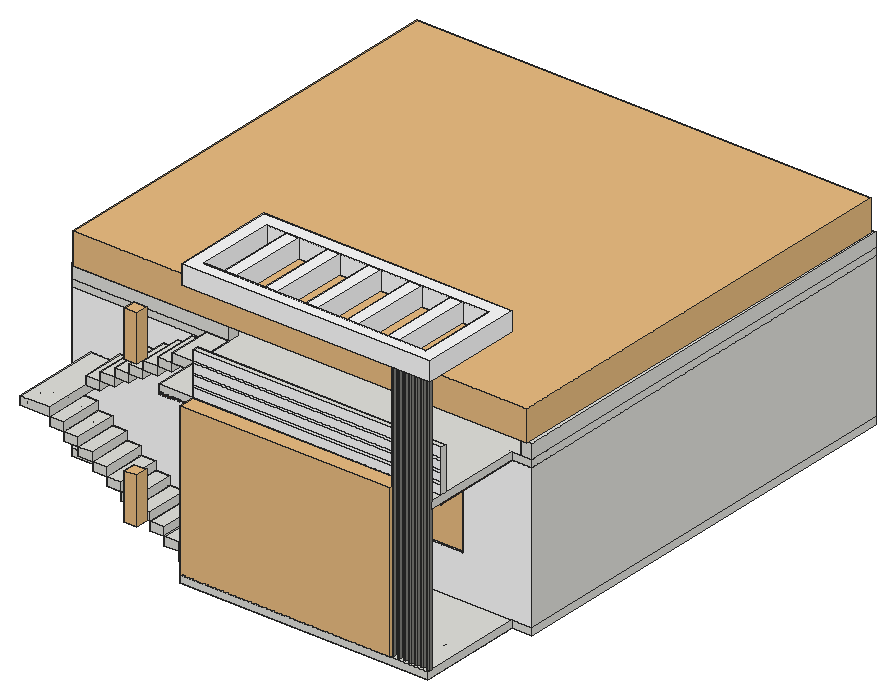
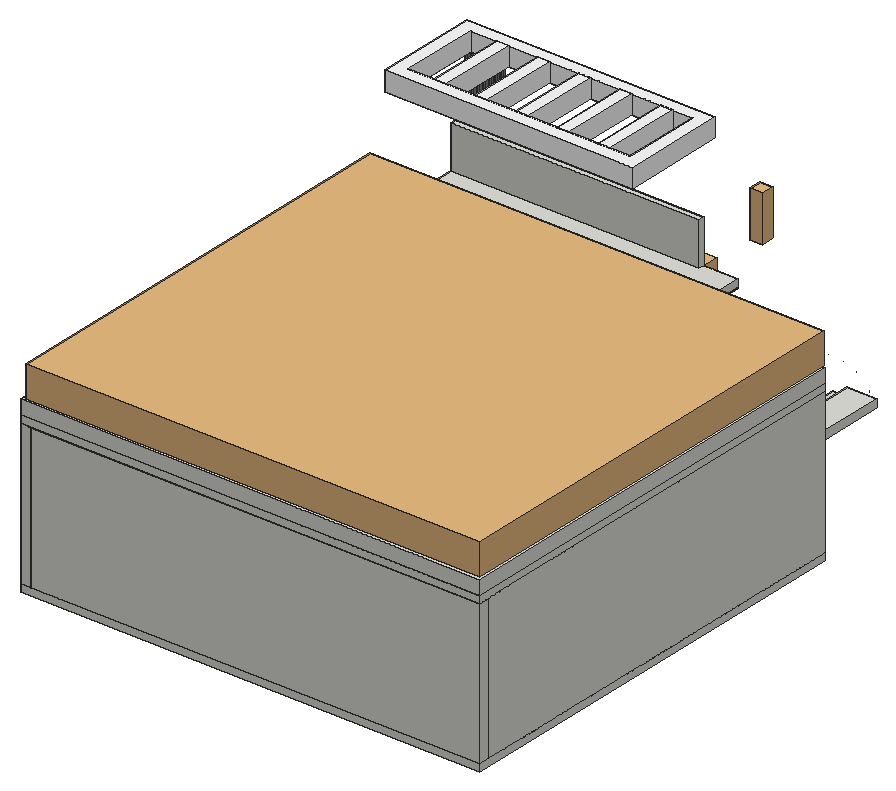
# SketchUp Ruby script. Lengths in inches.
U = 1.inch
M = Sketchup.active_model
def pt(a) = Geom::Point3d.new(a.map { |v| v * U })
def face(e, loops, mat)
  f = e.add_face(loops[0].map { |a| pt(a) })
  loops[1..].each { |l| e.add_face(l.map { |a| pt(a) }).erase! }
  f.material = f.back_material = mat if mat
  f
end
# faces: each face lists its corners as indices into pts; further lists are holes
def faces(e, pts, list, mat = nil) = list.each { |f| face(e, (f[0].is_a?(Array) ? f : [f]).map { |l| l.map { |i| pts[i] } }, mat) }
# xy, xz, yz: faces in a plane at the given z, y or x. An outline is a flat list of corners, or four numbers for a rectangle; further outlines are holes
def ring(l) = l.size == 4 ? [[l[0], l[1]], [l[2], l[1]], [l[2], l[3]], [l[0], l[3]]] : l.each_slice(2).to_a
def flat(e, list, mat, &to3) = list.each { |f| face(e, (f[0].is_a?(Array) ? f : [f]).map { |l| ring(l).map { |u, v| to3.(u, v) } }, mat) }
def xy(e, z, list, mat = nil) = flat(e, list, mat) { |x, y| [x, y, z] }
def xz(e, y, list, mat = nil) = flat(e, list, mat) { |x, z| [x, y, z] }
def yz(e, x, list, mat = nil) = flat(e, list, mat) { |y, z| [x, y, z] }
def lines(e, pts, list) = list.each { |a, b| e.add_line(pt(pts[a]), pt(pts[b])) }
# prism: a flat outline (further loops are holes) pulled along v
def prism(e, loops, v, mat = nil)
  f = face(e, loops, mat); d = Geom::Vector3d.new(v.map { |x| x * U })
  f.pushpull(f.normal.samedirection?(d) ? d.length : -d.length)
end
def box(e, o, s, mat = nil) = prism(e, [[o, [o[0] + s[0], o[1], o[2]], [o[0] + s[0], o[1] + s[1], o[2]], [o[0], o[1] + s[1], o[2]]]], [0, 0, s[2]], mat)
def at(x, y, z, deg = 0) = Geom::Transformation.translation(pt([x, y, z])) * Geom::Transformation.rotation(ORIGIN, Z_AXIS, deg.degrees)
def axes(o, x, y, z) = Geom::Transformation.new([*x, 0, *y, 0, *z, 0, *pt(o).to_a, 1])
def part(name) = M.definitions.add(name)
# library, detail: a bought-in or finely detailed component or shape, given as its bounding box
def library(name, o, s) = part(name).tap { |d| box(d.entities, o, s) }
def detail(e, o, s) = box(e.add_group.entities, o, s)
def put(e, d, t, mat = nil) = e.add_instance(d, t).tap { |i| i.material = mat if mat }
def group(e, t, mat = nil) = e.add_group.tap { |g| g.transformation = t; g.material = mat if mat }.entities
root = M.entities
M.materials.add("Carpaint Black Matte 1.5cm").color = [255, 255, 255]
M.materials.add("Ecorel - epc61025 33.57cm").color = [255, 255, 255]
M.materials.add("Iron Rough 15cm").color = [129, 129, 125]
M.materials.add("Leather Brown Alcantara 004 9.18cm").color = [255, 255, 255]
M.materials.add("Pp-1846-msg 17.72cm").color = [255, 255, 255]
M.materials.add("Wood Mahogany 33-46 100cm").color = [84, 42, 21]
M.materials.add("XPS Yellow SSS 1.51cm\#2").color = [255, 255, 255]
c1 = part("Group231\#1")
box(c1.entities,[-103.625,-42.25,0],[2,84.5,2])
c2 = part("Group232\#1")
box(c2.entities,[-99.625,-42.25,0],[2,84.5,2])
c3 = part("Group233\#1")
box(c3.entities,[-95.625,-42.25,0],[2,84.5,2])
c4 = part("Group234\#1")
box(c4.entities,[-91.625,-42.25,0],[2,84.5,2])
c5 = part("Group235\#1")
box(c5.entities,[-87.625,-42.25,0],[2,84.5,2])
c6 = part("Group236\#1")
box(c6.entities,[-83.625,-42.25,0],[2,84.5,2])
c7 = part("Group237\#1")
box(c7.entities,[-79.625,-42.25,0],[2,84.5,2])
c8 = part("Group238\#1")
box(c8.entities,[-75.625,-42.25,0],[2,84.5,2])
c9 = part("Group239\#1")
box(c9.entities,[-71.625,-42.25,0],[2,84.5,2])
c10 = part("Group240\#1")
box(c10.entities,[-67.625,-42.25,0],[2,84.5,2])
c11 = part("Group241\#1")
box(c11.entities,[-63.625,-42.25,0],[2,84.5,2])
c12 = part("Group242\#1")
box(c12.entities,[-59.625,-42.25,0],[2,84.5,2])
c13 = part("Group243\#1")
box(c13.entities,[-55.625,-42.25,0],[2,84.5,2])
c14 = part("Group244\#1")
box(c14.entities,[-51.625,-42.25,0],[2,84.5,2])
c15 = part("Group245\#1")
box(c15.entities,[-47.625,-42.25,0],[2,84.5,2])
c16 = part("Group246\#1")
box(c16.entities,[-43.625,-42.25,0],[2,84.5,2])
c17 = part("Group247\#1")
box(c17.entities,[-39.625,-42.25,0],[2,84.5,2])
c18 = part("Group248\#1")
box(c18.entities,[-35.625,-42.25,0],[2,84.5,2])
c19 = part("Group249\#1")
box(c19.entities,[-31.625,-42.25,0],[2,84.5,2])
c20 = part("Group250\#1")
box(c20.entities,[-27.625,-42.25,0],[2,84.5,2])
c21 = part("Group251\#1")
box(c21.entities,[-23.625,-42.25,0],[2,84.5,2])
c22 = part("Group252\#1")
box(c22.entities,[-19.625,-42.25,0],[2,84.5,2])
c23 = part("Group253\#1")
box(c23.entities,[-15.625,-42.25,0],[2,84.5,2])
c24 = part("Group254\#1")
box(c24.entities,[-11.625,-42.25,0],[2,84.5,2])
c25 = part("Group255\#1")
box(c25.entities,[-7.625,-42.25,0],[2,84.5,2])
c26 = part("Group256\#1")
box(c26.entities,[-3.625,-42.25,0],[2,84.5,2])
c27 = part("Group257\#1")
xy(c27.entities,0,[[0.375,-42.25,0.375,-42.1,2.375,-41.28,2.375,-42.25],[0.375,-42.1,0.375,42.25,2.375,42.25,2.375,-41.28]])
xy(c27.entities,2,[[0.375,-42.25,2.375,42.25]])
xz(c27.entities,-42.25,[[0.375,0,2.375,2]])
xz(c27.entities,42.25,[[0.375,0,2.375,2]])
yz(c27.entities,0.375,[[-42.25,0,42.25,2]])
yz(c27.entities,2.375,[[-42.25,0,42.25,2]])
c28 = part("Group258\#1")
xy(c28.entities,0,[[4.375,-42.25,4.375,-40.47,6.375,-39.65,6.375,-42.25],[4.375,-40.47,4.375,42.25,6.375,42.25,6.375,-39.65]])
xy(c28.entities,2,[[4.375,-42.25,6.375,42.25]])
xz(c28.entities,-42.25,[[4.375,0,6.375,2]])
xz(c28.entities,42.25,[[4.375,0,6.375,2]])
yz(c28.entities,4.375,[[-42.25,0,42.25,2]])
yz(c28.entities,6.375,[[-42.25,0,42.25,2]])
c29 = part("Group259\#1")
xy(c29.entities,0,[[8.375,-42.25,8.375,-38.84,10.375,-38.02,10.375,-42.25],[8.375,-38.84,8.375,42.25,10.375,42.25,10.375,-38.02]])
xy(c29.entities,2,[[8.375,-42.25,10.375,42.25]])
xz(c29.entities,-42.25,[[8.375,0,10.375,2]])
xz(c29.entities,42.25,[[8.375,0,10.375,2]])
yz(c29.entities,8.375,[[-42.25,0,42.25,2]])
yz(c29.entities,10.375,[[-42.25,0,42.25,2]])
c30 = part("Group260\#1")
xy(c30.entities,0,[[12.375,-42.25,12.375,-37.2,14.375,-36.39,14.375,-42.25],[12.375,-37.2,12.375,42.25,14.375,42.25,14.375,-36.39]])
xy(c30.entities,2,[[12.375,-42.25,14.375,42.25]])
xz(c30.entities,-42.25,[[12.375,0,14.375,2]])
xz(c30.entities,42.25,[[12.375,0,14.375,2]])
yz(c30.entities,12.375,[[-42.25,0,42.25,2]])
yz(c30.entities,14.375,[[-42.25,0,42.25,2]])
c31 = part("Group261\#1")
xy(c31.entities,0,[[16.375,-42.25,16.375,-35.57,18.375,-34.76,18.375,-42.25],[16.375,-35.57,16.375,42.25,18.375,42.25,18.375,-34.76]])
xy(c31.entities,2,[[16.375,-42.25,18.375,42.25]])
xz(c31.entities,-42.25,[[16.375,0,18.375,2]])
xz(c31.entities,42.25,[[16.375,0,18.375,2]])
yz(c31.entities,16.375,[[-42.25,0,42.25,2]])
yz(c31.entities,18.375,[[-42.25,0,42.25,2]])
c32 = part("Group262\#1")
xy(c32.entities,0,[[20.375,-42.25,20.375,-33.94,22.375,-33.13,22.375,-42.25],[20.375,-33.94,20.375,42.25,22.375,42.25,22.375,-33.13]])
xy(c32.entities,2,[[20.375,-42.25,22.375,42.25]])
xz(c32.entities,-42.25,[[20.375,0,22.375,2]])
xz(c32.entities,42.25,[[20.375,0,22.375,2]])
yz(c32.entities,20.375,[[-42.25,0,42.25,2]])
yz(c32.entities,22.375,[[-42.25,0,42.25,2]])
c33 = part("Group263\#1")
xy(c33.entities,0,[[24.375,-42.25,24.375,-32.3125,26.375,-31.5,26.375,-42.25],[24.375,-32.3125,24.375,42.25,26.375,42.25,26.375,-31.5]])
xy(c33.entities,2,[[24.375,-42.25,26.375,42.25]])
xz(c33.entities,-42.25,[[24.375,0,26.375,2]])
xz(c33.entities,42.25,[[24.375,0,26.375,2]])
yz(c33.entities,24.375,[[-42.25,0,42.25,2]])
yz(c33.entities,26.375,[[-42.25,0,42.25,2]])
c34 = part("Group264\#1")
xy(c34.entities,0,[[28.375,-42.25,28.375,-30.68,30.375,-29.87,30.375,-42.25],[28.375,-30.68,28.375,42.25,30.375,42.25,30.375,-29.87]])
xy(c34.entities,2,[[28.375,-42.25,30.375,42.25]])
xz(c34.entities,-42.25,[[28.375,0,30.375,2]])
xz(c34.entities,42.25,[[28.375,0,30.375,2]])
yz(c34.entities,28.375,[[-42.25,0,42.25,2]])
yz(c34.entities,30.375,[[-42.25,0,42.25,2]])
c35 = part("Group265\#1")
xy(c35.entities,0,[[32.375,-42.25,32.375,-29.05,34.375,-28.24,34.375,-42.25],[32.375,-29.05,32.375,42.25,34.375,42.25,34.375,-28.24]])
xy(c35.entities,2,[[32.375,-42.25,34.375,42.25]])
xz(c35.entities,-42.25,[[32.375,0,34.375,2]])
xz(c35.entities,42.25,[[32.375,0,34.375,2]])
yz(c35.entities,32.375,[[-42.25,0,42.25,2]])
yz(c35.entities,34.375,[[-42.25,0,42.25,2]])
c36 = part("Group266\#1")
xy(c36.entities,0,[[36.375,-42.25,36.375,-27.42,38.375,-26.6,38.375,-42.25],[36.375,-27.42,36.375,42.25,38.375,42.25,38.375,-26.6]])
xy(c36.entities,2,[[36.375,-42.25,38.375,42.25]])
xz(c36.entities,-42.25,[[36.375,0,38.375,2]])
xz(c36.entities,42.25,[[36.375,0,38.375,2]])
yz(c36.entities,36.375,[[-42.25,0,42.25,2]])
yz(c36.entities,38.375,[[-42.25,0,42.25,2]])
c37 = part("Group267\#1")
xy(c37.entities,0,[[40.375,-42.25,40.375,-25.79,42.375,-24.97,42.375,-42.25],[40.375,-25.79,40.375,42.25,42.375,42.25,42.375,-24.97]])
xy(c37.entities,2,[[40.375,-42.25,42.375,42.25]])
xz(c37.entities,-42.25,[[40.375,0,42.375,2]])
xz(c37.entities,42.25,[[40.375,0,42.375,2]])
yz(c37.entities,40.375,[[-42.25,0,42.25,2]])
yz(c37.entities,42.375,[[-42.25,0,42.25,2]])
c38 = part("Group268\#1")
xy(c38.entities,0,[[44.375,-42.25,44.375,-24.16,46.375,-23.34,46.375,-42.25],[44.375,-24.16,44.375,42.25,46.375,42.25,46.375,-23.34]])
xy(c38.entities,2,[[44.375,-42.25,46.375,42.25]])
xz(c38.entities,-42.25,[[44.375,0,46.375,2]])
xz(c38.entities,42.25,[[44.375,0,46.375,2]])
yz(c38.entities,44.375,[[-42.25,0,42.25,2]])
yz(c38.entities,46.375,[[-42.25,0,42.25,2]])
c39 = part("Group269\#1")
xy(c39.entities,0,[[48.375,-42.25,48.375,-22.53,50.375,-21.71,50.375,-42.25],[48.375,-22.53,48.375,42.25,50.375,42.25,50.375,-21.71]])
xy(c39.entities,2,[[48.375,-42.25,50.375,42.25]])
xz(c39.entities,-42.25,[[48.375,0,50.375,2]])
xz(c39.entities,42.25,[[48.375,0,50.375,2]])
yz(c39.entities,48.375,[[-42.25,0,42.25,2]])
yz(c39.entities,50.375,[[-42.25,0,42.25,2]])
c40 = part("Group270\#1")
xy(c40.entities,0,[[52.375,-42.25,52.375,-20.9,54.375,-20.08,54.375,-42.25],[52.375,-20.9,52.375,42.25,54.375,42.25,54.375,-20.08]])
xy(c40.entities,2,[[52.375,-42.25,54.375,42.25]])
xz(c40.entities,-42.25,[[52.375,0,54.375,2]])
xz(c40.entities,42.25,[[52.375,0,54.375,2]])
yz(c40.entities,52.375,[[-42.25,0,42.25,2]])
yz(c40.entities,54.375,[[-42.25,0,42.25,2]])
c41 = part("Group271\#1")
xy(c41.entities,0,[[56.375,-42.25,56.375,-19.27,58.375,-18.45,58.375,-42.25],[56.375,-19.27,56.375,42.25,58.375,42.25,58.375,-18.45]])
xy(c41.entities,2,[[56.375,-42.25,58.375,42.25]])
xz(c41.entities,-42.25,[[56.375,0,58.375,2]])
xz(c41.entities,42.25,[[56.375,0,58.375,2]])
yz(c41.entities,56.375,[[-42.25,0,42.25,2]])
yz(c41.entities,58.375,[[-42.25,0,42.25,2]])
c42 = part("Group272\#1")
xy(c42.entities,0,[[60.375,-42.25,60.375,-17.63,62.375,-16.82,62.375,-42.25],[60.375,-17.63,60.375,42.25,62.375,42.25,62.375,-16.82]])
xy(c42.entities,2,[[60.375,-42.25,62.375,42.25]])
xz(c42.entities,-42.25,[[60.375,0,62.375,2]])
xz(c42.entities,42.25,[[60.375,0,62.375,2]])
yz(c42.entities,60.375,[[-42.25,0,42.25,2]])
yz(c42.entities,62.375,[[-42.25,0,42.25,2]])
c43 = part("Group273\#1")
xy(c43.entities,0,[[64.375,-42.25,64.375,-16,66.375,-15.1875,66.375,-42.25],[64.375,-16,64.375,42.25,66.375,42.25,66.375,-15.1875]])
xy(c43.entities,2,[[64.375,-42.25,66.375,42.25]])
xz(c43.entities,-42.25,[[64.375,0,66.375,2]])
xz(c43.entities,42.25,[[64.375,0,66.375,2]])
yz(c43.entities,64.375,[[-42.25,0,42.25,2]])
yz(c43.entities,66.375,[[-42.25,0,42.25,2]])
c44 = part("Group274\#1")
xy(c44.entities,0,[[68.375,-42.25,68.375,-14.37,70.375,-13.56,70.375,-42.25],[68.375,-14.37,68.375,42.25,70.375,42.25,70.375,-13.56]])
xy(c44.entities,2,[[68.375,-42.25,70.375,42.25]])
xz(c44.entities,-42.25,[[68.375,0,70.375,2]])
xz(c44.entities,42.25,[[68.375,0,70.375,2]])
yz(c44.entities,68.375,[[-42.25,0,42.25,2]])
yz(c44.entities,70.375,[[-42.25,0,42.25,2]])
c45 = part("Group275\#1")
xy(c45.entities,0,[[72.375,-42.25,72.375,-12.74,74.375,-11.93,74.375,-42.25],[72.375,-12.74,72.375,42.25,74.375,42.25,74.375,-11.93]])
xy(c45.entities,2,[[72.375,-42.25,74.375,42.25]])
xz(c45.entities,-42.25,[[72.375,0,74.375,2]])
xz(c45.entities,42.25,[[72.375,0,74.375,2]])
yz(c45.entities,72.375,[[-42.25,0,42.25,2]])
yz(c45.entities,74.375,[[-42.25,0,42.25,2]])
c46 = part("Group276\#1")
xy(c46.entities,0,[[76.375,-42.25,76.375,-11.11,78.375,-10.3,78.375,-42.25],[76.375,-11.11,76.375,42.25,78.375,42.25,78.375,-10.3]])
xy(c46.entities,2,[[76.375,-42.25,78.375,42.25]])
xz(c46.entities,-42.25,[[76.375,0,78.375,2]])
xz(c46.entities,42.25,[[76.375,0,78.375,2]])
yz(c46.entities,76.375,[[-42.25,0,42.25,2]])
yz(c46.entities,78.375,[[-42.25,0,42.25,2]])
c47 = part("Group277\#1")
xy(c47.entities,0,[[80.375,-42.25,80.375,-9.48,82.375,-8.66,82.375,-42.25],[80.375,-9.48,80.375,42.25,82.375,42.25,82.375,-8.66]])
xy(c47.entities,2,[[80.375,-42.25,82.375,42.25]])
xz(c47.entities,-42.25,[[80.375,0,82.375,2]])
xz(c47.entities,42.25,[[80.375,0,82.375,2]])
yz(c47.entities,80.375,[[-42.25,0,42.25,2]])
yz(c47.entities,82.375,[[-42.25,0,42.25,2]])
c48 = part("Group278\#1")
xy(c48.entities,0,[[84.375,-42.25,84.375,-7.85,86.375,-7.03,86.375,-42.25],[84.375,-7.85,84.375,42.25,86.375,42.25,86.375,-7.03]])
xy(c48.entities,2,[[84.375,-42.25,86.375,42.25]])
xz(c48.entities,-42.25,[[84.375,0,86.375,2]])
xz(c48.entities,42.25,[[84.375,0,86.375,2]])
yz(c48.entities,84.375,[[-42.25,0,42.25,2]])
yz(c48.entities,86.375,[[-42.25,0,42.25,2]])
c49 = part("Group279\#1")
xy(c49.entities,0,[[88.375,-42.25,88.375,-6.22,90.375,-5.4,90.375,-42.25],[88.375,-6.22,88.375,42.25,90.375,42.25,90.375,-5.4]])
xy(c49.entities,2,[[88.375,-42.25,90.375,42.25]])
xz(c49.entities,-42.25,[[88.375,0,90.375,2]])
xz(c49.entities,42.25,[[88.375,0,90.375,2]])
yz(c49.entities,88.375,[[-42.25,0,42.25,2]])
yz(c49.entities,90.375,[[-42.25,0,42.25,2]])
c50 = part("Group280\#1")
xy(c50.entities,0,[[92.375,-42.25,92.375,-4.59,94.375,-3.77,94.375,-42.25],[92.375,-4.59,92.375,42.25,94.375,42.25,94.375,-3.77]])
xy(c50.entities,2,[[92.375,-42.25,94.375,42.25]])
xz(c50.entities,-42.25,[[92.375,0,94.375,2]])
xz(c50.entities,42.25,[[92.375,0,94.375,2]])
yz(c50.entities,92.375,[[-42.25,0,42.25,2]])
yz(c50.entities,94.375,[[-42.25,0,42.25,2]])
c51 = part("Group281\#1")
xy(c51.entities,0,[[96.375,-42.25,96.375,-2.96,98.375,-2.14,98.375,-42.25],[96.375,-2.96,96.375,42.25,98.375,42.25,98.375,-2.14]])
xy(c51.entities,2,[[96.375,-42.25,98.375,42.25]])
xz(c51.entities,-42.25,[[96.375,0,98.375,2]])
xz(c51.entities,42.25,[[96.375,0,98.375,2]])
yz(c51.entities,96.375,[[-42.25,0,42.25,2]])
yz(c51.entities,98.375,[[-42.25,0,42.25,2]])
c52 = part("Group282\#1")
xy(c52.entities,0,[[100.375,-42.25,100.375,-1.33,102.375,-0.51,102.375,-42.25],[100.375,-1.33,100.375,42.25,102.375,42.25,102.375,-0.51]])
xy(c52.entities,2,[[100.375,-42.25,102.375,42.25]])
xz(c52.entities,-42.25,[[100.375,0,102.375,2]])
xz(c52.entities,42.25,[[100.375,0,102.375,2]])
yz(c52.entities,100.375,[[-42.25,0,42.25,2]])
yz(c52.entities,102.375,[[-42.25,0,42.25,2]])
c53 = part("Group229\#1")
put(c53.entities,c1,at(0,0,0))
put(c53.entities,c2,at(0,0,0))
put(c53.entities,c3,at(0,0,0))
put(c53.entities,c4,at(0,0,0))
put(c53.entities,c5,at(0,0,0))
put(c53.entities,c6,at(0,0,0))
put(c53.entities,c7,at(0,0,0))
put(c53.entities,c8,at(0,0,0))
put(c53.entities,c9,at(0,0,0))
put(c53.entities,c10,at(0,0,0))
put(c53.entities,c11,at(0,0,0))
put(c53.entities,c12,at(0,0,0))
put(c53.entities,c13,at(0,0,0))
put(c53.entities,c14,at(0,0,0))
put(c53.entities,c15,at(0,0,0))
put(c53.entities,c16,at(0,0,0))
put(c53.entities,c17,at(0,0,0))
put(c53.entities,c18,at(0,0,0))
put(c53.entities,c19,at(0,0,0))
put(c53.entities,c20,at(0,0,0))
put(c53.entities,c21,at(0,0,0))
put(c53.entities,c22,at(0,0,0))
put(c53.entities,c23,at(0,0,0))
put(c53.entities,c24,at(0,0,0))
put(c53.entities,c25,at(0,0,0))
put(c53.entities,c26,at(0,0,0))
put(c53.entities,c27,at(0,0,0))
put(c53.entities,c28,at(0,0,0))
put(c53.entities,c29,at(0,0,0))
put(c53.entities,c30,at(0,0,0))
put(c53.entities,c31,at(0,0,0))
put(c53.entities,c32,at(0,0,0))
put(c53.entities,c33,at(0,0,0))
put(c53.entities,c34,at(0,0,0))
put(c53.entities,c35,at(0,0,0))
put(c53.entities,c36,at(0,0,0))
put(c53.entities,c37,at(0,0,0))
put(c53.entities,c38,at(0,0,0))
put(c53.entities,c39,at(0,0,0))
put(c53.entities,c40,at(0,0,0))
put(c53.entities,c41,at(0,0,0))
put(c53.entities,c42,at(0,0,0))
put(c53.entities,c43,at(0,0,0))
put(c53.entities,c44,at(0,0,0))
put(c53.entities,c45,at(0,0,0))
put(c53.entities,c46,at(0,0,0))
put(c53.entities,c47,at(0,0,0))
put(c53.entities,c48,at(0,0,0))
put(c53.entities,c49,at(0,0,0))
put(c53.entities,c50,at(0,0,0))
put(c53.entities,c51,at(0,0,0))
put(c53.entities,c52,at(0,0,0))
c54 = library("Group\#18",[0,-1.6875,-0.04],[175.25,13.6875,126.04])
c55 = library("Window Crafter Sliding",[0,-0.55,0],[60,4.49,60])
c56 = library("Door 243 065",[-19.36,-2.49,0],[38.72,4.98,81.96])
c57 = part("Stair tread")
box(c57.entities,[0,0,0],[12,36,7])
c58 = part("Stair tread \#1")
box(c58.entities,[0,0,0],[19.0625,36,7])
c59 = part("Stair landing")
box(c59.entities,[-12.25,0,0],[24.25,74,7])
c60 = part("Group188\#1")
box(c60.entities,[-17.75,-79.99,0],[2,215.82,2])
c61 = part("Group189\#1")
box(c61.entities,[-12.75,-79.99,0],[2,215.82,2])
c62 = part("Group190\#1")
box(c62.entities,[-7.75,-79.99,0],[2,215.82,2])
c63 = part("Group191\#1")
box(c63.entities,[-2.75,-79.99,0],[2,215.82,2])
c64 = part("Group192\#1")
box(c64.entities,[2.25,-79.99,0],[2,215.82,2])
c65 = part("Group193\#1")
box(c65.entities,[7.25,-79.99,0],[2,215.82,2])
c66 = part("Group194\#1")
box(c66.entities,[12.25,-79.99,0],[2,215.82,2])
c67 = part("Group186\#1")
put(c67.entities,c60,at(0,0,0))
put(c67.entities,c61,at(0,0,0))
put(c67.entities,c62,at(0,0,0))
put(c67.entities,c63,at(0,0,0))
put(c67.entities,c64,at(0,0,0))
put(c67.entities,c65,at(0,0,0))
put(c67.entities,c66,at(0,0,0))
c68 = library("Group\#39",[0,0,0],[129.13,3.15,25.98])
c69 = library("Group\#44",[0,0,0],[10.21,10.4,38.37])
c70 = library("Tlon Light 650 Ceiling 152 007",[-12.8,-12.8,-3.78],[25.6,25.6,3.58])
c71 = part("Group284\#1")
box(c71.entities,[-118.09,-37,0],[2,74,2])
c72 = part("Group285\#1")
box(c72.entities,[-114.09,-37,0],[2,74,2])
c73 = part("Group286\#1")
box(c73.entities,[-110.09,-37,0],[2,74,2])
c74 = part("Group287\#1")
box(c74.entities,[-106.09,-37,0],[2,74,2])
c75 = part("Group288\#1")
box(c75.entities,[-102.09,-37,0],[2,74,2])
c76 = part("Group289\#1")
box(c76.entities,[-98.09,-37,0],[2,74,2])
c77 = part("Group290\#1")
box(c77.entities,[-94.09,-37,0],[2,74,2])
c78 = part("Group291\#1")
box(c78.entities,[-90.09,-37,0],[2,74,2])
c79 = part("Group292\#1")
box(c79.entities,[-86.09,-37,0],[2,74,2])
c80 = part("Group293\#1")
box(c80.entities,[-82.09,-37,0],[2,74,2])
c81 = part("Group294\#1")
box(c81.entities,[-78.09,-37,0],[2,74,2])
c82 = part("Group295\#1")
box(c82.entities,[-74.09,-37,0],[2,74,2])
c83 = part("Group296\#1")
box(c83.entities,[-70.09,-37,0],[2,74,2])
c84 = part("Group297\#1")
box(c84.entities,[-66.09,-37,0],[2,74,2])
c85 = part("Group298\#1")
box(c85.entities,[-62.09,-37,0],[2,74,2])
c86 = part("Group299\#1")
box(c86.entities,[-58.09,-37,0],[2,74,2])
c87 = part("Group300\#1")
box(c87.entities,[-54.09,-37,0],[2,74,2])
c88 = part("Group301\#1")
box(c88.entities,[-50.09,-37,0],[2,74,2])
c89 = part("Group302\#1")
box(c89.entities,[-46.09,-37,0],[2,74,2])
c90 = part("Group303\#1")
box(c90.entities,[-42.09,-37,0],[2,74,2])
c91 = part("Group304\#1")
box(c91.entities,[-38.09,-37,0],[2,74,2])
c92 = part("Group305\#1")
box(c92.entities,[-34.09,-37,0],[2,74,2])
c93 = part("Group306\#1")
box(c93.entities,[-30.09,-37,0],[2,74,2])
c94 = part("Group307\#1")
box(c94.entities,[-26.09,-37,0],[2,74,2])
c95 = part("Group308\#1")
box(c95.entities,[-22.09,-37,0],[2,74,2])
c96 = part("Group309\#1")
box(c96.entities,[-18.09,-37,0],[2,74,2])
c97 = part("Group310\#1")
box(c97.entities,[-14.09,-37,0],[2,74,2])
c98 = part("Group311\#1")
box(c98.entities,[-10.09,-37,0],[2,74,2])
c99 = part("Group312\#1")
box(c99.entities,[-6.09,-37,0],[2,74,2])
c100 = part("Group313\#1")
box(c100.entities,[-2.09,-37,0],[2,74,2])
c101 = part("Group314\#1")
box(c101.entities,[1.91,-37,0],[2,74,2])
c102 = part("Group315\#1")
box(c102.entities,[5.91,-37,0],[2,74,2])
c103 = part("Group316\#1")
box(c103.entities,[9.91,-37,0],[2,74,2])
c104 = part("Group317\#1")
box(c104.entities,[13.91,-37,0],[2,74,2])
c105 = part("Group318\#1")
box(c105.entities,[17.91,-37,0],[2,74,2])
c106 = part("Group319\#1")
box(c106.entities,[21.91,-37,0],[2,74,2])
c107 = part("Group320\#1")
box(c107.entities,[25.91,-37,0],[2,74,2])
c108 = part("Group321\#1")
box(c108.entities,[29.91,-37,0],[2,74,2])
c109 = part("Group322\#1")
box(c109.entities,[33.91,-37,0],[2,74,2])
c110 = part("Group323\#1")
box(c110.entities,[37.91,-37,0],[2,74,2])
c111 = part("Group324\#1")
box(c111.entities,[41.91,-37,0],[2,74,2])
c112 = part("Group325\#1")
box(c112.entities,[45.91,-37,0],[2,74,2])
c113 = part("Group326\#1")
box(c113.entities,[49.91,-37,0],[2,74,2])
c114 = part("Group327\#1")
box(c114.entities,[53.91,-37,0],[2,74,2])
c115 = part("Group328\#1")
box(c115.entities,[57.91,-37,0],[2,74,2])
c116 = part("Group329\#1")
box(c116.entities,[61.91,-37,0],[2,74,2])
c117 = part("Group330\#1")
box(c117.entities,[65.91,-37,0],[2,74,2])
c118 = part("Group331\#1")
box(c118.entities,[69.91,-37,0],[2,74,2])
c119 = part("Group332\#1")
box(c119.entities,[73.91,-37,0],[2,74,2])
c120 = part("Group333\#1")
box(c120.entities,[77.91,-37,0],[2,74,2])
c121 = part("Group334\#1")
box(c121.entities,[81.91,-37,0],[2,74,2])
c122 = part("Group335\#1")
box(c122.entities,[85.91,-37,0],[2,74,2])
c123 = part("Group336\#1")
box(c123.entities,[89.91,-37,0],[2,74,2])
c124 = part("Group337\#1")
box(c124.entities,[93.91,-37,0],[2,74,2])
c125 = part("Group338\#1")
box(c125.entities,[97.91,-37,0],[2,74,2])
c126 = part("Group339\#1")
box(c126.entities,[101.91,-37,0],[2,74,2])
c127 = part("Group340\#1")
box(c127.entities,[105.91,-37,0],[2,74,2])
c128 = part("Group341\#1")
box(c128.entities,[109.91,-37,0],[2,74,2])
c129 = part("Group342\#1")
box(c129.entities,[113.91,-37,0],[2,74,2])
c130 = part("Group343\#1")
xy(c130.entities,0,[[117.91,-37,118.09,37]])
xy(c130.entities,2,[[117.91,-37,118.09,37]])
yz(c130.entities,117.91,[[-37,0,37,2]])
c131 = part("Group282\#2")
put(c131.entities,c71,at(0,0,0))
put(c131.entities,c72,at(0,0,0))
put(c131.entities,c73,at(0,0,0))
put(c131.entities,c74,at(0,0,0))
put(c131.entities,c75,at(0,0,0))
put(c131.entities,c76,at(0,0,0))
put(c131.entities,c77,at(0,0,0))
put(c131.entities,c78,at(0,0,0))
put(c131.entities,c79,at(0,0,0))
put(c131.entities,c80,at(0,0,0))
put(c131.entities,c81,at(0,0,0))
put(c131.entities,c82,at(0,0,0))
put(c131.entities,c83,at(0,0,0))
put(c131.entities,c84,at(0,0,0))
put(c131.entities,c85,at(0,0,0))
put(c131.entities,c86,at(0,0,0))
put(c131.entities,c87,at(0,0,0))
put(c131.entities,c88,at(0,0,0))
put(c131.entities,c89,at(0,0,0))
put(c131.entities,c90,at(0,0,0))
put(c131.entities,c91,at(0,0,0))
put(c131.entities,c92,at(0,0,0))
put(c131.entities,c93,at(0,0,0))
put(c131.entities,c94,at(0,0,0))
put(c131.entities,c95,at(0,0,0))
put(c131.entities,c96,at(0,0,0))
put(c131.entities,c97,at(0,0,0))
put(c131.entities,c98,at(0,0,0))
put(c131.entities,c99,at(0,0,0))
put(c131.entities,c100,at(0,0,0))
put(c131.entities,c101,at(0,0,0))
put(c131.entities,c102,at(0,0,0))
put(c131.entities,c103,at(0,0,0))
put(c131.entities,c104,at(0,0,0))
put(c131.entities,c105,at(0,0,0))
put(c131.entities,c106,at(0,0,0))
put(c131.entities,c107,at(0,0,0))
put(c131.entities,c108,at(0,0,0))
put(c131.entities,c109,at(0,0,0))
put(c131.entities,c110,at(0,0,0))
put(c131.entities,c111,at(0,0,0))
put(c131.entities,c112,at(0,0,0))
put(c131.entities,c113,at(0,0,0))
put(c131.entities,c114,at(0,0,0))
put(c131.entities,c115,at(0,0,0))
put(c131.entities,c116,at(0,0,0))
put(c131.entities,c117,at(0,0,0))
put(c131.entities,c118,at(0,0,0))
put(c131.entities,c119,at(0,0,0))
put(c131.entities,c120,at(0,0,0))
put(c131.entities,c121,at(0,0,0))
put(c131.entities,c122,at(0,0,0))
put(c131.entities,c123,at(0,0,0))
put(c131.entities,c124,at(0,0,0))
put(c131.entities,c125,at(0,0,0))
put(c131.entities,c126,at(0,0,0))
put(c131.entities,c127,at(0,0,0))
put(c131.entities,c128,at(0,0,0))
put(c131.entities,c129,at(0,0,0))
put(c131.entities,c130,at(0,0,0))
c132 = library("Group\#46",[0,0,0],[378.52,359.23,25.98])
c133 = part("Component\#5")
box(c133.entities,[0,-65.71,0],[10.1875,65.71,15.8125])
p = [[2295.1875,-533,944.94],[2295.1875,-536,944.94],[1790.2,-533,944.94],[1790.2,-536,944.94],[754.01,394.47,340.74],[754.01,394.47,339.65],
  [743.375,394.47,348.15],[743.375,394.47,347.69],[732.74,394.47,350.77],[732.74,394.47,350.69],[720.1,394.47,350.29],[720.1,394.47,350.08],
  [709.47,394.47,346.27],[709.47,394.47,345.65],[698.83,394.47,336.13],[698.83,394.47,334.51],[833.45,388.26,252],[833.45,472.76,252],
  [1040.7,472.76,252],[1040.7,388.26,252],[1040.7,398.76,378],[804.51,398.76,378],[804.51,472.76,378],[1040.7,472.76,378]]
lines(root,p,[[0,1],[2,3],[4,5],[6,7],[8,9],[10,11],[12,13],[14,15],[16,17],[17,18],[18,19],[19,16],
  [20,21],[21,22],[22,23],[23,20]])
put(root,c53,at(937.07,430.51,251),"Wood Mahogany 33-46 100cm")
g1 = group(root,at(672.95,472.76,252))
prism(g1,[[[367.75,-87.6875,0],[160.5,-87.6875,0],[160.5,-74,0],[160.5,-38,0],[131.5625,-38,0],[131.5625,0,0],[0,0,0],[0,360,0],[384,360,0],[384,0,0],[367.75,0,0]]],[0,0,6])
put(root,c54,at(833.45,386.76,258))
g2 = group(root,at(672.95,472.76,258))
put(g2,c55,at(266.5625,2.73,36))
put(g2,c56,axes([198.48,4.93,0],[1,0,0],[0,1,0],[0,0,1.17128]))
g3 = group(g2,at(0,0,0))
xy(g3,0,[[179.1875,0,218.1875,9],[9,9,102,129],[106.5,9,226.5,129],[231,9,375,129],[9,133.5,102,262.5],
  [106.5,133.5,226.5,262.5],[231,133.5,375,262.5],[9,267,102,351],[106.5,267,226.5,351],[231,267,375,351]])
xy(g3,36,[[266.5625,0,326.5625,9]])
xy(g3,96,[[179.1875,0,218.1875,9],[266.5625,0,326.5625,9]])
xy(g3,120,[[[0,0,384,0,384,360,375,360,375,267,231,267,231,351,375,351,375,360,0,360,0,351,226.5,351,226.5,267,106.5,267,106.5,351,102,351,102,267,9,267,9,262.5,102,262.5,102,133.5,9,133.5,9,351,0,351],[106.5,9,106.5,129,226.5,129,226.5,9,231,9,231,129,375,129,375,9],[231,133.5,375,262.5],[106.5,133.5,226.5,262.5],[9,9,102,129]]])
xz(g3,0,[[[0,0,179.1875,0,179.1875,96,218.1875,96,218.1875,0,384,0,384,120,0,120],[266.5625,36,326.5625,96]]],"Pp-1846-msg 17.72cm")
xz(g3,9,[[9,0,102,120],[106.5,0,106.5,120,226.5,120,226.5,0,218.1875,0,218.1875,96,179.1875,96,179.1875,0],[226.5,0,231,120],[[231,0,375,120],[266.5625,36,326.5625,96]]])
xz(g3,129,[[9,0,102,120],[106.5,0,226.5,120],[231,0,375,120]])
xz(g3,133.5,[[9,0,102,120],[106.5,0,226.5,120],[231,0,375,120]])
xz(g3,262.5,[[9,0,102,120],[106.5,0,226.5,120],[231,0,375,120]])
xz(g3,267,[[9,0,102,120],[106.5,0,226.5,120],[231,0,375,120]])
xz(g3,351,[[0,0,9,120],[9,0,102,120],[102,0,106.5,120],[106.5,0,226.5,120],[231,0,375,120]])
xz(g3,360,[[0,0,375,120],[375,0,384,120]])
yz(g3,0,[[0,0,351,120],[351,0,360,120]])
yz(g3,9,[[9,0,129,120],[133.5,0,262.5,120],[262.5,0,267,120],[267,0,351,120]])
yz(g3,102,[[9,0,129,120],[133.5,0,262.5,120],[267,0,351,120]])
yz(g3,106.5,[[9,0,129,120],[133.5,0,262.5,120],[267,0,351,120]])
yz(g3,179.1875,[[0,0,9,96]])
yz(g3,218.1875,[[0,0,9,96]])
yz(g3,226.5,[[9,0,129,120],[133.5,0,262.5,120],[267,0,351,120]])
yz(g3,231,[[9,0,129,120],[133.5,0,262.5,120],[267,0,351,120]])
yz(g3,266.5625,[[0,36,9,96]])
yz(g3,326.5625,[[0,36,9,96]])
yz(g3,375,[[9,0,129,120],[133.5,0,262.5,120],[267,0,351,120],[351,0,360,120]])
yz(g3,384,[[0,0,360,120]])
g4 = group(root,at(677.45,398.76,258))
put(g4,c57,at(36,38,77))
put(g4,c57,at(132,0,7))
put(g4,c57,at(108,0,21))
put(g4,c57,at(120,0,14))
put(g4,c57,at(144,0,0))
put(g4,c57,at(60,38,91))
put(g4,c57,at(84,38,105))
put(g4,c57,at(96,38,112))
put(g4,c57,at(48,38,84))
put(g4,c58,at(108,38,119))
put(g4,c57,at(72,38,98))
put(g4,c57,at(48,0,56))
put(g4,c57,at(60,0,49))
put(g4,c59,at(24,0,70))
put(g4,c57,at(36,0,63))
put(g4,c57,at(84,0,35))
put(g4,c57,at(96,0,28))
put(g4,c57,at(72,0,42))
g5 = group(root,at(856.47,390.88,258))
xy(g5,0,[[0,1.625,0,7.875,125.45,7.875,125.45,1.625,94.41,1.625,94.41,2.625,93.78,2.625,93.78,1.625,63.04,1.625,63.04,2.625,62.41,2.625,62.41,1.625,31.68,1.625,31.68,2.625,31.05,2.625,31.05,1.625]],"Leather Brown Alcantara 004 9.18cm")
xy(g5,24,[[0,1.625,31.05,1.625,31.05,2.625,31.68,2.625,31.68,1.625,62.41,1.625,62.41,2.625,63.04,2.625,63.04,1.625,93.78,1.625,93.78,2.625,94.41,2.625,94.41,1.625,125.45,1.625,125.45,7.875,0,7.875]],"Leather Brown Alcantara 004 9.18cm")
xz(g5,1.625,[[0,0,31.05,24],[31.68,0,62.41,24],[63.04,0,93.78,24],[94.41,0,125.45,24]],"Leather Brown Alcantara 004 9.18cm")
xz(g5,2.625,[[31.05,0,31.68,24],[62.41,0,63.04,24],[93.78,0,94.41,24]],"Carpaint Black Matte 1.5cm")
xz(g5,7.875,[[0,0,125.45,24]],"Leather Brown Alcantara 004 9.18cm")
yz(g5,0,[[1.625,0,7.875,24]],"Leather Brown Alcantara 004 9.18cm")
yz(g5,31.05,[[1.625,0,2.625,24]],"Carpaint Black Matte 1.5cm")
yz(g5,31.68,[[1.625,0,2.625,24]],"Carpaint Black Matte 1.5cm")
yz(g5,62.41,[[1.625,0,2.625,24]],"Carpaint Black Matte 1.5cm")
yz(g5,63.04,[[1.625,0,2.625,24]],"Carpaint Black Matte 1.5cm")
yz(g5,93.78,[[1.625,0,2.625,24]],"Carpaint Black Matte 1.5cm")
yz(g5,94.41,[[1.625,0,2.625,24]],"Carpaint Black Matte 1.5cm")
yz(g5,125.45,[[1.625,0,7.875,24]],"Leather Brown Alcantara 004 9.18cm")
put(root,c67,axes([1026.45,388.76,338.04],[1,0,0],[0,0,1],[0,-1,0]),"Iron Rough 15cm")
put(root,c68,at(854.5,394.06,282))
put(root,c69,at(793.58,376.76,287.01))
put(root,c70,axes([918.65,433.24,376.2],[0.58,0,0],[0,0.58,0],[0,0,0.58]))
put(root,c131,at(922.61,435.76,377),"Wood Mahogany 33-46 100cm")
g6 = group(root,at(672.95,472.76,378))
xy(g6,0,[[335.75,-84,335.75,-74,131.5625,-74,131.5625,0,0,0,0,360,384,360,384,0,367.75,0,367.75,-84]])
xy(g6,6,[[335.75,-84,367.75,-84,367.75,0,375,0,375,351,9,351,9,9,131.5625,9,131.5625,-74,335.75,-74]])
xz(g6,-84,[[335.75,0,367.75,6]])
xz(g6,-74,[[131.5625,0,309.3125,6],[309.3125,0,335.75,6]])
xz(g6,0,[[0,0,131.5625,6],[367.75,0,384,6]])
xz(g6,360,[[0,0,384,6]])
yz(g6,0,[[0,0,360,6]])
yz(g6,131.5625,[[-74,0,0,6]])
yz(g6,335.75,[[-84,0,-74,6]])
yz(g6,367.75,[[-84,0,0,6]])
yz(g6,384,[[0,0,360,6]])
p = [[365.55,0,0.01],[365.55,0,6]]
lines(g6,p,[[0,1]])
g7 = group(g6,at(0,0,6))
xy(g7,0,[[0,0,0,360,384,360,384,0,375,0,375,351,9,351,9,9,131.5625,9,131.5625,0]])
xy(g7,12,[[[0,0,131.5625,0,131.5625,9,9,9,9,351,375,351,375,0,384,0,384,360,0,360],[4.3125,4.3125,4.3125,355.6875,379.6875,355.6875,379.6875,4.3125,379.3125,4.3125,379.3125,355.3125,4.6875,355.3125,4.6875,4.6875,127.25,4.6875,127.25,4.3125]],[4.3125,4.3125,127.25,4.3125,127.25,4.6875,4.6875,4.6875,4.6875,355.3125,379.3125,355.3125,379.3125,4.3125,379.6875,4.3125,379.6875,355.6875,4.3125,355.6875]])
xz(g7,0,[[0,0,131.5625,12],[375,0,384,12]])
xz(g7,9,[[9,0,131.5625,12]])
xz(g7,351,[[9,0,375,12]])
xz(g7,360,[[0,0,384,12]])
yz(g7,0,[[0,0,360,12]])
yz(g7,9,[[9,0,351,12]])
yz(g7,131.5625,[[0,0,9,12]])
yz(g7,375,[[0,0,351,12]])
yz(g7,384,[[0,0,360,12]])
g8 = group(root,at(833.45,398.76,384))
xy(g8,0,[[0,0,207.25,4.5]])
xy(g8,36,[[0,0,207.25,4.5]])
xz(g8,0,[[0,8,207.25,10],[0,17,207.25,19],[0,26,207.25,28]],"Carpaint Black Matte 1.5cm")
xz(g8,0,[[0,0,207.25,8],[0,10,207.25,17],[0,19,207.25,26],[0,28,207.25,36]],"XPS Yellow SSS 1.51cm\#2")
xz(g8,4.5,[[0,0,207.25,36]])
yz(g8,0,[[0,0,4.5,36]])
yz(g8,207.25,[[0,0,4.5,36]])
put(root,c132,at(675.6875,470.79,396))
put(root,c69,at(793.58,376.76,408.63))
g9 = group(root,at(833.45,403.26,473.875),"Ecorel - epc61025 33.57cm")
prism(g9,[[[207.25,69.5,0],[207.25,-16.5,0],[0,-16.5,0],[0,69.5,0]],[[10.93,-7.14,0],[196.33,-7.14,0],[196.33,58.57,0],[27.65,58.57,0],[10.93,58.57,0]]],[0,0,15.8125])
put(g9,c133,at(27.65,58.57,0))
put(g9,c133,at(164.46,58.57,0))
put(g9,c133,at(61.85,58.57,0))
put(g9,c133,at(96.05,58.57,0))
put(g9,c133,at(130.26,58.57,0))
